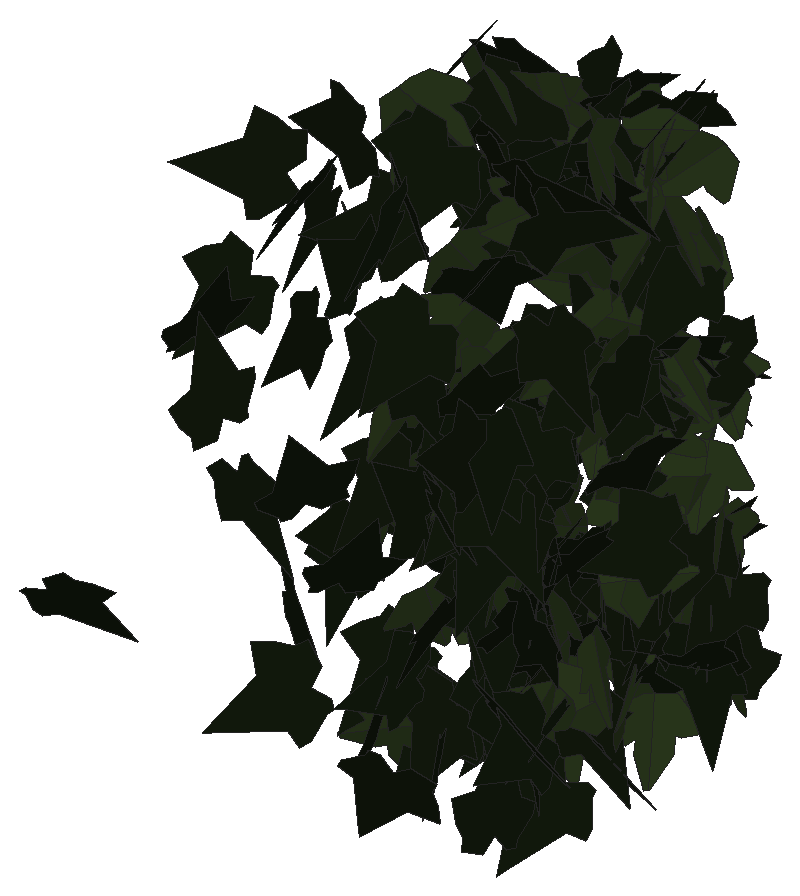
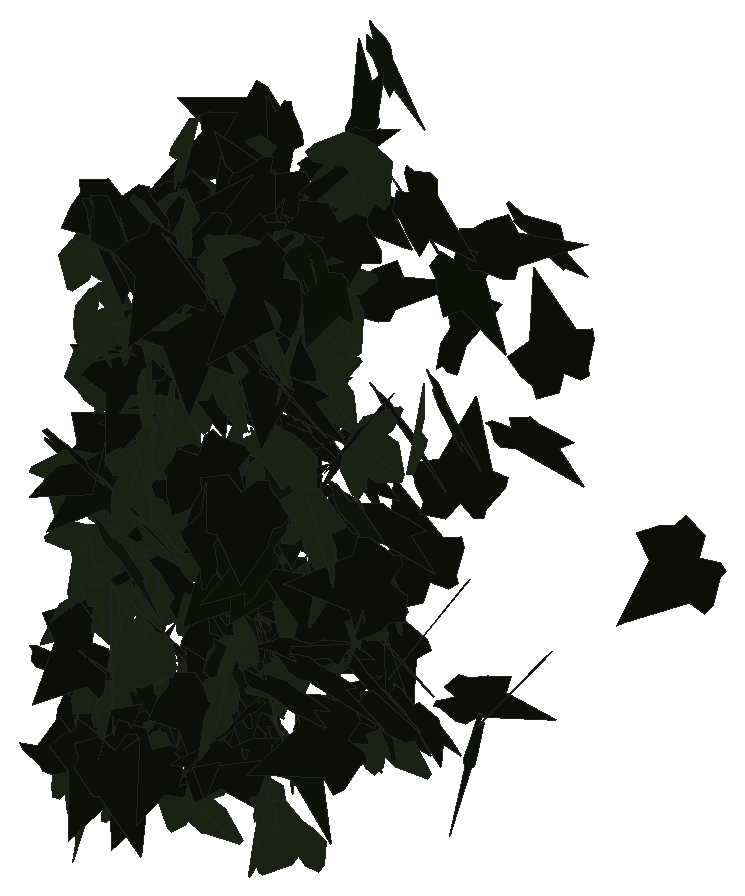
# SketchUp Ruby script. Lengths in inches.
U = 1.inch
M = Sketchup.active_model
def pt(a) = Geom::Point3d.new(a.map { |v| v * U })
def face(e, loops, mat)
  f = e.add_face(loops[0].map { |a| pt(a) })
  loops[1..].each { |l| e.add_face(l.map { |a| pt(a) }).erase! }
  f.material = f.back_material = mat if mat
  f
end
# faces: each face lists its corners as indices into pts; further lists are holes
def faces(e, pts, list, mat = nil) = list.each { |f| face(e, (f[0].is_a?(Array) ? f : [f]).map { |l| l.map { |i| pts[i] } }, mat) }
# xy, xz, yz: faces in a plane at the given z, y or x. An outline is a flat list of corners, or four numbers for a rectangle; further outlines are holes
def ring(l) = l.size == 4 ? [[l[0], l[1]], [l[2], l[1]], [l[2], l[3]], [l[0], l[3]]] : l.each_slice(2).to_a
def flat(e, list, mat, &to3) = list.each { |f| face(e, (f[0].is_a?(Array) ? f : [f]).map { |l| ring(l).map { |u, v| to3.(u, v) } }, mat) }
def xy(e, z, list, mat = nil) = flat(e, list, mat) { |x, y| [x, y, z] }
def xz(e, y, list, mat = nil) = flat(e, list, mat) { |x, z| [x, y, z] }
def yz(e, x, list, mat = nil) = flat(e, list, mat) { |y, z| [x, y, z] }
def lines(e, pts, list) = list.each { |a, b| e.add_line(pt(pts[a]), pt(pts[b])) }
# prism: a flat outline (further loops are holes) pulled along v
def prism(e, loops, v, mat = nil)
  f = face(e, loops, mat); d = Geom::Vector3d.new(v.map { |x| x * U })
  f.pushpull(f.normal.samedirection?(d) ? d.length : -d.length)
end
def box(e, o, s, mat = nil) = prism(e, [[o, [o[0] + s[0], o[1], o[2]], [o[0] + s[0], o[1] + s[1], o[2]], [o[0], o[1] + s[1], o[2]]]], [0, 0, s[2]], mat)
def at(x, y, z, deg = 0) = Geom::Transformation.translation(pt([x, y, z])) * Geom::Transformation.rotation(ORIGIN, Z_AXIS, deg.degrees)
def axes(o, x, y, z) = Geom::Transformation.new([*x, 0, *y, 0, *z, 0, *pt(o).to_a, 1])
def part(name) = M.definitions.add(name)
# library, detail: a bought-in or finely detailed component or shape, given as its bounding box
def library(name, o, s) = part(name).tap { |d| box(d.entities, o, s) }
def detail(e, o, s) = box(e.add_group.entities, o, s)
def put(e, d, t, mat = nil) = e.add_instance(d, t).tap { |i| i.material = mat if mat }
def group(e, t, mat = nil) = e.add_group.tap { |g| g.transformation = t; g.material = mat if mat }.entities
root = M.entities
M.materials.add("efeu1").color = [18, 25, 13]
M.materials.add("efeu2").color = [43, 57, 29]
c1 = part("ivyleaf_9")
p = [[1.54,2.16,1.25],[1.36,2.04,1.19],[-0.21,0.99,0.68],[-0.71,1.11,0.82],[-0.85,0.86,0.67],[-0.8,0.17,0.21],
  [-0.9,-0.01,0.1],[-0.67,-0.16,-0.02],[-0.08,-0.08,-0.05],[-0.03,-0.6,-0.4],[0.65,-0.88,-0.66],[0.83,-0.6,-0.49],
  [1.29,-0.42,-0.43],[1.8125,-0.07,-0.26],[1.21,0.44,0.15]]
faces(c1.entities,p,[[0,1,2,3,4,5,6,7,8,9,10,11,12,13,14]],"efeu1")
c2 = part("ivyleaf_10")
p = [[0,0.5,-0.03],[-0.0625,2.02,-0.43],[-0.19,2.01,-0.46],[-0.54,1.05,-0.29],[-0.52,0.625,-0.18],[-0.83,0.76,-0.28],
  [-1.16,0.64,-0.33],[-1.15,0.33,-0.24],[-0.77,-0.39,0.02],[-0.3,-0.51,0.16],[0.04,-0.48,0.23],[-0.02,2.01,-0.4375],
  [-0.06,2.01,-0.43],[0.04,-0.49,0.23],[0.67,-0.49,0.14],[1.38,0.36,-0.2],[1.375,0.51,-0.24],[0.81,0.65,-0.19],
  [0.62,0.59,-0.15],[0.6,1.09,-0.28],[0.5,1.23,-0.31]]
faces(c2.entities,p,[[0,1,2,3,4,5,6,7,8,9,10],[11,12,0,13,14,15,16,17,18,19,20]],"efeu2")
put(root,c1,axes([1.91,221.53,235.64],[0.22863,-0.36807,-0.09829],[-0.00412,0.10612,-0.43871],[0.41039,0.20612,0.05036]))
put(root,c1,axes([2.04,217.83,235.76],[0.42687,0.15912,0.09116],[0.08714,0.03428,-0.44312],[-0.17578,0.4034,0.0017]))
put(root,c1,axes([2.52,220.89,238.83],[-0.44623,-0.13584,0.00812],[-0.00782,-0.00297,-0.45233],[0.14674,-0.41324,0.00058]))
put(root,c1,axes([2.8,221.32,234.46],[0.2674,-0.1092,-0.35421],[-0.3342,0.14231,-0.28141],[0.1937,0.39629,0.00346]))
put(root,c1,axes([2.92,221.94,239.62],[-0.37271,0.12519,-0.2427],[0.23278,-0.08994,-0.38167],[-0.16618,-0.40677,0.0097]))
put(root,c1,axes([2.97,219.37,238.9],[0.24821,0.31767,0.19593],[-0.11941,-0.15254,0.40777],[0.38059,-0.25504,0.00015]))
put(root,c1,axes([3.48,220.34,240.84],[-0.23642,-0.04216,0.38848],[-0.38822,-0.10298,-0.23117],[0.11877,-0.42053,0.01766]))
put(root,c2,axes([3.16,222.16,238.78],[-0.2934,0.28026,0.19972],[0.14683,-0.13566,0.40592],[0.33626,0.30377,-0.00299]))
put(root,c1,axes([3.2,222.06,235.05],[-0.37672,-0.07268,-0.25952],[0.27137,0.01248,-0.36907],[0.07176,-0.4287,0.03325]))
put(root,c1,axes([3.34,222.51,237.02],[0.11116,0.25592,-0.34981],[0.04678,0.33797,0.28123],[0.45406,-0.09748,0.05666]))
put(root,c1,axes([3.74,220.55,240.65],[-0.23139,0.32472,-0.20241],[0.08986,-0.17778,-0.40373],[-0.39887,-0.22842,0.02647]))
put(root,c2,axes([3.6,222.6875,236.56],[-0.12476,0.29797,-0.30692],[0.07464,-0.2884,-0.33097],[-0.44674,-0.1314,0.03042]))
put(root,c1,axes([4.09,222.42,235.67],[-0.38619,0.23182,0.21706],[-0.18444,0.11449,-0.45042],[-0.25853,-0.42797,-0.00292]))
put(root,c1,axes([3.99,220.17,234.11],[-0.36444,-0.1518,0.23787],[-0.22521,-0.09397,-0.38482],[0.19282,-0.39667,0.00013]))
put(root,c1,axes([3.94,223.46,236.03],[-0.49598,-0.06285,-0.00765],[0.01361,-0.04677,-0.49762],[0.06184,-0.49382,0.0481]))
put(root,c1,axes([3.72,221.51,235.45],[0.19024,-0.34359,-0.20836],[0.09783,-0.17871,0.40156],[-0.41827,-0.19807,-0.00085]))
put(root,c1,axes([4.09,222.76,241.36],[0.04322,0.36416,0.24392],[-0.01197,0.23632,-0.37964],[-0.46765,0.02761,0.03226]))
put(root,c1,axes([4.35,220.7,241.51],[-0.11201,0.06327,-0.4344],[-0.43613,-0.14117,0.08204],[-0.13401,0.40656,0.09609]))
put(root,c2,axes([4.21,223,237.99],[-0.44215,0.05122,0.22777],[-0.23326,-0.07694,-0.43551],[-0.00956,-0.49138,0.09194]))
put(root,c1,axes([3.7,222.91,234.78],[0.4087,0.06535,0.21249],[0.21981,0.02155,-0.3992],[-0.07321,0.42952,-0.0123]))
put(root,c2,axes([4.15,223.84,234.18],[0.0767,-0.37169,-0.32552],[0.00816,0.33032,-0.37526],[0.49402,0.05225,0.05673]))
put(root,c2,axes([4.13,222.73,236.99],[-0.1661,0.42601,-0.2023],[-0.0532,-0.23004,-0.44074],[-0.4686,-0.12489,0.12174]))
put(root,c2,axes([3.875,223.66,233.75],[0.38828,0.08163,0.30426],[0.28914,0.09934,-0.39563],[-0.12505,0.48318,0.02994]))
put(root,c1,axes([3.79,222.85,236.47],[0.32966,0.15313,-0.28023],[0.25976,0.12146,0.35516],[0.21109,-0.38862,0.00059]))
put(root,c1,axes([4.18,219.93,236.82],[0.28208,0.17465,0.31287],[-0.26574,-0.17317,0.32672],[0.26557,-0.35879,-0.00539]))
put(root,c1,axes([4.35,223.59,235.6875],[-0.46956,-0.13976,-0.09989],[0.11476,-0.03884,-0.4851],[0.12784,-0.4785,0.06855]))
put(root,c1,axes([4.08,223.11,236.13],[-0.19881,-0.41807,-0.18891],[0.22689,0.08934,-0.43651],[0.39874,-0.25929,0.15419]))
put(root,c2,axes([4.25,221.4,236.43],[0.40162,-0.29312,0.05273],[0.04132,-0.03283,-0.49721],[0.29494,0.40374,-0.00215]))
put(root,c1,axes([4.47,221.03,238.55],[-0.46847,0.10262,-0.14145],[0.14112,-0.01654,-0.47939],[-0.10307,-0.48908,-0.01347]))
put(root,c1,axes([4.625,221.57,237.26],[-0.23945,0.33896,0.16501],[-0.10902,0.12342,-0.42091],[-0.38922,-0.2431,0.01638]))
put(root,c2,axes([4.63,223.45,240.74],[0.17537,-0.15369,-0.4423],[-0.33914,0.28395,-0.23314],[0.32284,0.38177,-0.00465]))
put(root,c1,axes([4.29,219.94,239.28],[0.00885,-0.14754,-0.4255],[0.29714,-0.31517,0.12393],[-0.36379,-0.26101,0.09087]))
put(root,c2,axes([4.44,222.98,240.4],[-0.23147,0.3678,0.0931],[-0.04652,0.07851,-0.44271],[-0.40616,-0.2186,-0.00235]))
put(root,c1,axes([4.58,221.36,234.32],[-0.4209,-0.19256,0.01681],[-0.01592,-0.00666,-0.45209],[0.20808,-0.39,-0.00058]))
put(root,c1,axes([4.71,221.2,240.11],[-0.24158,-0.08892,0.37683],[-0.34095,-0.18003,-0.24863],[0.21473,-0.38589,0.02916]))
put(root,c2,axes([4.87,220.82,233.63],[-0.18329,-0.03834,0.41464],[-0.41276,-0.11405,-0.1806],[0.12942,-0.41803,0.01124]))
put(root,c2,axes([4.73,222.09,240.66],[-0.30498,-0.30563,0.25215],[-0.17014,-0.18634,-0.43166],[0.35782,-0.3491,0.00966]))
put(root,c2,axes([4.68,222.72,241.46],[-0.45211,0.17823,0.11761],[-0.13564,-0.02701,-0.48049],[-0.16493,-0.46637,0.07277]))
put(root,c1,axes([4.72,221.13,236.91],[-0.44715,-0.13343,-0.002],[0.00182,0.00104,-0.4524],[0.14411,-0.41403,-0.00049]))
put(root,c1,axes([4.38,223.36,241.43],[0.49307,0.08084,-0.01864],[-0.01555,-0.02027,-0.49935],[-0.08149,0.49301,-0.01747]))
put(root,c1,axes([4.86,217.5,239.3],[-0.44645,0.07294,-0.11869],[-0.12498,0.00024,0.4361],[0.07601,0.42884,0.01994]))
put(root,c1,axes([4.47,220.24,235.71],[0.33519,0.27585,0.13483],[-0.10596,-0.08477,0.43184],[0.31166,-0.3255,0.0018]))
put(root,c1,axes([4.88,222.96,239.58],[-0.47782,-0.14516,0.02476],[-0.02349,-0.00787,-0.49939],[0.14537,-0.4784,0.00071]))
put(root,c2,axes([4.71,221.27,237.97],[-0.04403,-0.33624,0.36743],[0.0614,-0.36971,-0.33097],[0.49426,0.01598,0.07385]))
put(root,c1,axes([4.74,221.73,241.37],[0.29999,0.28944,-0.17494],[-0.1364,-0.11182,-0.417],[-0.33483,0.30487,0.01313]))
put(root,c1,axes([5.03,223.16,240.08],[-0.45458,0.19879,0.06197],[-0.05888,0.02002,-0.49612],[-0.19973,-0.45835,0.00521]))
put(root,c2,axes([4.81,222.58,236.24],[0.00958,-0.13557,0.42977],[-0.00025,-0.41333,-0.14101],[0.4697,0.00254,-0.00884]))
put(root,c1,axes([4.69,220.49,233.45],[0.0285,0.30612,0.32024],[-0.06786,-0.30256,0.31841],[0.464,-0.06305,0.0269]))
put(root,c1,axes([4.54,223.35,237.43],[0.41422,-0.2796,-0.01559],[0.0049,0.03508,-0.49874],[0.27999,0.41303,0.03181]))
put(root,c1,axes([4.88,222.89,240.1],[0.22329,0.36146,-0.13082],[-0.0561,-0.11514,-0.43291],[-0.40952,0.21286,-0.01202]))
put(root,c1,axes([4.68,221.28,238.26],[0.25092,-0.38907,-0.18885],[-0.08712,0.16839,-0.46266],[0.42361,0.26509,0.01672]))
put(root,c2,axes([4.93,223.63,235.875],[-0.28292,0.30763,0.16758],[-0.10194,0.13117,-0.42002],[-0.36094,-0.27818,-0.01273]))
put(root,c2,axes([5.05,223.58,235.17],[-0.00151,0.18181,0.41099],[-0.18354,0.36355,-0.17458],[-0.43246,-0.15492,0.07266]))
put(root,c1,axes([5.24,222.14,237.59],[-0.20989,0.36517,0.13994],[-0.09032,0.1077,-0.4296],[-0.41049,-0.21041,0.02297]))
put(root,c1,axes([5.18,223.64,234.54],[-0.12312,0.28985,-0.31582],[-0.03229,-0.31948,-0.30546],[-0.45223,-0.0561,0.10779]))
put(root,c1,axes([5.22,221.98,233.77],[-0.21082,0.3885,-0.01428],[0.00384,-0.01358,-0.45216],[-0.41982,-0.19522,0.00303]))
put(root,c1,axes([5.32,219.46,240.38],[-0.15963,0.24995,0.33685],[-0.1875,0.27352,-0.30191],[-0.40009,-0.2279,0.00709]))
put(root,c1,axes([5.14,223.17,237.93],[0.24959,0.27867,-0.25082],[-0.19043,-0.16636,-0.37564],[-0.34951,0.28964,0.02556]))
put(root,c2,axes([5.03,220.85,241.36],[-0.04364,0.36744,0.33628],[-0.02524,0.3355,-0.36987],[-0.49745,-0.04926,-0.01074]))
put(root,c2,axes([5.25,221.63,238.98],[-0.23345,-0.26805,0.27643],[-0.16532,-0.21774,-0.35783],[0.37267,-0.2645,0.01443]))
put(root,c1,axes([5.32,221.51,236.8125],[-0.18239,0.08143,-0.40822],[-0.37409,0.18478,0.19485],[0.21795,0.38529,-0.00717]))
put(root,c2,axes([5.08,221.1,235.35],[-0.19617,-0.36509,-0.15754],[0.07411,0.13505,-0.42408],[0.4204,-0.19416,0.00125]))
put(root,c1,axes([4.84,223.78,234.625],[0.05969,-0.39616,-0.29916],[0.10371,0.30462,-0.38269],[0.48547,-0.01637,0.11853]))
put(root,c2,axes([4.92,221.07,242.01],[-0.32586,-0.19515,-0.32516],[0.31837,0.09216,-0.37437],[0.20605,-0.45103,0.06419]))
put(root,c2,axes([5.1,221.63,239.79],[-0.15753,-0.31569,-0.27178],[0.13259,0.23098,-0.36147],[0.42227,-0.1903,0.01211]))
put(root,c1,axes([5.07,222.93,241.33],[-0.15838,-0.47345,0.02749],[0.00782,-0.03158,-0.49894],[0.47419,-0.15762,0.0174]))
put(root,c2,axes([5.12,222.11,234.875],[0.01544,-0.03948,0.45029],[-0.0226,0.43264,0.04175],[-0.469,-0.02215,0.01281]))
put(root,c2,axes([5.2,223.08,241.39],[-0.43157,-0.16053,-0.06391],[0.06028,0.0259,-0.44785],[0.17558,-0.40347,-0.00332]))
put(root,c1,axes([5.28,222.17,237.3],[-0.29199,0.16134,-0.31217],[0.19879,-0.25332,-0.31403],[-0.30973,-0.31468,0.09274]))
put(root,c1,axes([5,223.68,234.77],[0.11581,-0.48628,-0.01094],[-0.00117,0.01096,-0.49988],[0.4864,0.1158,0.0014]))
put(root,c1,axes([5.52,220.26,234.75],[-0.39538,0.21231,0.10463],[-0.10056,0.0399,-0.43996],[-0.23296,-0.37757,0.01234]))
put(root,c1,axes([5.43,222.83,235.12],[-0.0572,0.39888,0.17188],[-0.04856,0.1605,-0.41787],[-0.46377,-0.066,0.02256]))
put(root,c2,axes([5.5,223.28,239.78],[-0.36754,0.04791,0.27734],[-0.29262,-0.05965,-0.34845],[-0.00036,-0.42822,0.07956]))
put(root,c1,axes([5.375,221.24,233.83],[-0.42914,-0.17571,-0.02237],[0.01695,0.01767,-0.45173],[0.19043,-0.39754,-0.01019]))
put(root,c1,axes([5.08,221.12,241.73],[0.10355,-0.30357,-0.3083],[-0.01198,0.30202,-0.32538],[0.45809,0.07652,0.06118]))
put(root,c2,axes([5.54,223.85,233.78],[0.27974,0.06517,-0.35708],[-0.37518,0.00135,-0.27228],[-0.04121,0.43009,0.05496]))
put(root,c2,axes([5.15,222.24,238.15],[-0.3425,-0.12224,-0.28236],[0.28072,0.07982,-0.35313],[0.15685,-0.40977,0.01545]))
put(root,c1,axes([5.41,223.55,235.11],[0.14136,0.40087,-0.11102],[-0.03896,-0.10051,-0.43856],[-0.44633,0.13574,0.00312]))
put(root,c1,axes([5.71,220.22,237.03],[-0.26667,0.04086,-0.37002],[-0.38652,-0.01243,0.25683],[0.01408,0.4329,0.0423]))
put(root,c1,axes([5.73,222.35,240.36],[-0.34248,0.01657,-0.3092],[-0.32056,-0.05237,0.32621],[-0.02575,0.43152,0.05146]))
put(root,c1,axes([5.46,222.36,236.5625],[0.0923,0.33542,0.27401],[0.00335,0.26821,-0.35616],[-0.46063,0.06916,0.05231]))
put(root,c2,axes([5.11,223.04,241.14],[0.25833,0.09763,0.41681],[0.2611,0.34987,-0.24377],[-0.33925,0.3436,0.12978]))
put(root,c2,axes([5.22,222.18,233.77],[-0.13995,0.00138,-0.43186],[0.21283,-0.38269,-0.06527],[-0.39475,-0.20681,0.11791]))
put(root,c1,axes([5.47,223.36,237.21],[0.02405,-0.00157,0.4518],[0.10914,0.42308,-0.0038],[-0.45631,0.10111,0.0229]))
put(root,c1,axes([5.43,221.14,233.92],[-0.17635,-0.37956,0.14144],[-0.03736,-0.13299,-0.42923],[0.43384,-0.16574,0.02052]))
put(root,c1,axes([5.64,221.91,234.5],[0.04317,0.02492,0.44974],[-0.03082,0.43349,-0.02323],[-0.4668,-0.02631,0.04313]))
put(root,c1,axes([5.67,223.55,240.6],[0.29569,0.24859,-0.23823],[-0.19094,-0.14594,-0.38448],[-0.31117,0.32577,0.00955]))
put(root,c1,axes([5.75,220.3125,233.3],[0.00224,0.08388,0.4439],[-0.0298,0.426,-0.08693],[-0.46885,-0.02668,0.00764]))
put(root,c1,axes([5.88,222.49,236.2],[-0.1521,0.31082,0.28057],[-0.15134,0.23189,-0.35393],[-0.41794,-0.19709,0.02605]))
put(root,c1,axes([5.64,220.73,241.7],[-0.25264,-0.41632,0.11335],[-0.05836,-0.09718,-0.48698],[0.42751,-0.25929,0.00051]))
put(root,c1,axes([5.62,222.68,236.53],[0.18904,0.3088,0.26151],[0.05885,0.25351,-0.36324],[-0.42604,0.17204,0.06586]))
put(root,c1,axes([5.82,221.97,233.93],[-0.45898,0.00515,-0.09638],[0.09986,-0.01399,-0.44182],[-0.00865,-0.43474,0.01307]))
put(root,c1,axes([5.83,223.15,238.23],[-0.03944,0.27405,-0.34927],[0.01398,-0.33619,-0.28678],[-0.46793,-0.03314,0.02088]))
put(root,c1,axes([5.85,223.63,241.46],[-0.44152,0.10751,-0.10676],[0.11059,-0.01407,-0.43944],[-0.11637,-0.42127,-0.01256]))
put(root,c1,axes([5.62,222.42,237.76],[-0.06557,0.07534,-0.44107],[0.32515,-0.29889,-0.10004],[-0.33271,-0.30694,-0.01084]))
put(root,c1,axes([5.94,219.35,233.99],[0.21202,0.19552,-0.34876],[-0.26726,-0.2265,-0.288],[-0.323,0.31575,0.00937]))
put(root,c2,axes([5.84,222.24,234.9],[0.11751,-0.21115,0.379],[-0.10715,0.35294,0.24349],[-0.44207,-0.14168,0.04172]))
put(root,c1,axes([5.75,221.5,235.64],[-0.09905,-0.42373,0.03702],[0.01487,-0.03935,-0.45032],[0.459,-0.09016,0.02258]))
put(root,c1,axes([5.9375,221.5,236.93],[-0.23178,-0.30534,0.2324],[-0.11068,-0.2004,-0.38713],[0.39337,-0.23629,0.02801]))
put(root,c2,axes([5.83,223.47,234.96],[-0.20402,0.31232,-0.24609],[0.04111,-0.24682,-0.37041],[-0.42119,-0.17538,0.08305]))
put(root,c1,axes([5.87,223.59,241.29],[0.24421,0.36146,0.08973],[0.05361,0.07071,-0.44339],[-0.39774,0.23146,-0.00467]))
put(root,c2,axes([5.92,223.68,239.13],[-0.07899,0.33866,-0.27355],[-0.05702,-0.27191,-0.34883],[-0.45959,-0.02447,0.0903]))
put(root,c1,axes([5.57,221.46,236.79],[0.32295,-0.21634,0.23944],[0.20522,-0.1301,-0.3838],[0.27259,0.35425,0.00527]))
put(root,c1,axes([6.07,222.95,239.83],[0.0448,0.37122,-0.23185],[-0.04951,-0.21893,-0.38801],[-0.46503,0.05907,0.01897]))
put(root,c2,axes([5.93,223.7,240.36],[0.3925,0.23466,-0.04749],[-0.0377,-0.03011,-0.44985],[-0.25542,0.36504,-0.00658]))
put(root,c2,axes([6.06,223.76,239.08],[-0.45798,-0.09439,0.02312],[-0.02183,-0.01147,-0.45175],[0.10243,-0.42448,0.00706]))
put(root,c1,axes([5.98,224,234.26],[0.35182,0.27689,-0.08347],[-0.07877,-0.03801,-0.44424],[-0.30122,0.33334,0.01868]))
put(root,c2,axes([6.15,221.6,235.62],[0.1263,-0.0899,0.4256],[-0.26186,0.33198,0.14791],[-0.36904,-0.26634,0.0407]))
put(root,c1,axes([5.92,221.53,234.25],[-0.06738,-0.43043,0.00826],[-0.01371,-0.00618,-0.45216],[0.46474,-0.06259,-0.01214]))
put(root,c1,axes([6.3,221.89,234.61],[-0.36729,0.26784,0.04448],[-0.03577,0.02708,-0.45021],[-0.29074,-0.34169,-0.00081]))
put(root,c1,axes([6.17,220.1,236.01],[-0.20603,0.31121,-0.24606],[0.12032,-0.20907,-0.37943],[-0.40471,-0.22059,0.01247]))
put(root,c1,axes([6.375,221.54,238.93],[-0.37103,0.25783,0.0715],[-0.07274,0.02467,-0.44621],[-0.27885,-0.34949,0.02125]))
put(root,c1,axes([6.25,222.96,240],[-0.17382,0.3651,-0.18019],[0.06697,-0.16198,-0.41489],[-0.43129,-0.1723,0.0082]))
put(root,c2,axes([6.16,221.07,236.15],[0.21435,-0.36944,-0.25993],[-0.05958,0.26208,-0.42162],[0.44778,0.21173,0.06834]))
put(root,c1,axes([6.26,224.34,234.29],[0.01182,0.39579,-0.18737],[-0.02216,-0.17955,-0.41151],[-0.46913,0.01845,0.01472]))
put(root,c2,axes([6.18,223.77,239.4],[0.12172,-0.41864,-0.03702],[-0.01509,0.0331,-0.45085],[0.45351,0.11346,-0.00507]))
put(root,c1,axes([6.51,221.47,235.34],[-0.08811,0.14345,0.41858],[-0.39356,0.19059,-0.14747],[-0.24096,-0.36376,0.0878]))
put(root,c2,axes([6.18,221.41,237.46],[0.39399,-0.23174,-0.05139],[-0.04663,0.02419,-0.44946],[0.25162,0.36734,-0.00282]))
put(root,c1,axes([6.08,221.15,235.6875],[-0.28024,-0.2547,-0.24834],[0.18485,0.1665,-0.37814],[0.32864,-0.31085,0.00093]))
put(root,c2,axes([6.28,223.93,238.26],[0.03347,0.24344,0.37353],[-0.20083,0.33279,-0.2179],[-0.42339,-0.13861,0.13289]))
put(root,c1,axes([5.99,219.63,241.47],[-0.04265,-0.07224,0.44422],[0.13032,-0.41377,-0.06118],[0.44934,0.11314,0.05991]))
put(root,c1,axes([6.23,220.57,240.34],[0.25368,0.35829,-0.07838],[-0.04784,-0.06107,-0.44554],[-0.39252,0.23901,0.00365]))
put(root,c1,axes([6.49,221.55,236.6],[0.04493,0.03808,-0.44858],[-0.46759,-0.00278,-0.04369],[-0.00695,0.43332,0.03914]))
put(root,c2,axes([6.21,222.875,239.9375],[0.43386,0.15162,-0.07249],[-0.06944,-0.02703,-0.44655],[-0.16631,0.40682,-0.00266]))
put(root,c2,axes([6.07,224.02,235.88],[0.40696,0.13573,0.17653],[0.13001,0.15252,-0.40476],[-0.19543,0.38411,0.09834]))
put(root,c2,axes([6.28,222.04,237.1],[-0.46019,0.08632,0.01515],[0.01369,-0.01075,0.45207],[0.09355,0.42621,0.00834]))
put(root,c1,axes([6.44,220.74,240.49],[-0.14857,0.41252,0.01153],[-0.00475,0.01022,-0.45225],[-0.44566,-0.13764,0.00098]))
put(root,c1,axes([6.36,219.45,240.125],[-0.37965,-0.25422,0.03324],[-0.0309,-0.01497,-0.45115],[0.27499,-0.35266,-0.00481]))
put(root,c1,axes([6.46,220.5,237.43],[-0.46569,-0.05654,0.0102],[-0.01023,-0.00319,-0.45228],[0.06112,-0.4313,0.00201]))
put(root,c1,axes([6.17,219.9,237.54],[0.38728,-0.15387,-0.19994],[-0.17834,0.10167,-0.40496],[0.19728,0.39397,0.02641]))
put(root,c1,axes([6.38,221.74,241.25],[-0.01648,-0.10639,-0.43837],[0.11336,-0.4102,0.10372],[-0.45562,-0.09821,0.04166]))
put(root,c1,axes([6.19,223.73,234.41],[-0.07825,-0.45622,0.18906],[0.04707,-0.19744,-0.45695],[0.49159,-0.05371,0.07385]))
put(root,c1,axes([6.63,221.4,237.1],[-0.06836,0.27861,0.34114],[-0.23621,0.26472,-0.27773],[-0.4003,-0.20378,0.10563]))
put(root,c2,axes([6.4,221.16,236.24],[-0.05191,-0.43137,0.03008],[-0.00183,-0.02892,-0.4514],[0.46692,-0.04807,0.00157]))
put(root,c1,axes([6.64,223.85,237.02],[-0.239,0.31731,0.20687],[-0.13729,0.15368,-0.40205],[-0.38045,-0.25479,0.01513]))
put(root,c2,axes([6.54,221.72,233.75],[0.35586,-0.00558,-0.2953],[-0.30509,0.03835,-0.3417],[0.03159,0.43327,0.02644]))
put(root,c1,axes([6.4375,224.42,234.22],[0.10026,0.38725,0.18207],[0.03176,0.17291,-0.414],[-0.45788,0.09679,0.01115]))
put(root,c1,axes([6.5,221.77,234.89],[0.05489,0.41678,-0.11828],[-0.01427,-0.11296,-0.43666],[-0.46636,0.05251,-0.00056]))
put(root,c1,axes([6.58,223.67,238.74],[-0.41313,-0.16673,0.12781],[-0.10925,-0.07484,-0.43306],[0.1952,-0.39475,0.02812]))
put(root,c1,axes([6.53,218.6875,242.04],[-0.35881,0.21462,-0.1883],[0.16725,-0.09393,-0.41132],[-0.25297,-0.36652,-0.00485]))
put(root,c1,axes([6.2,221.125,240.85],[-0.2099,0.04791,0.40166],[0.40565,-0.08989,0.20817],[0.11,0.42291,-0.00125]))
put(root,c1,axes([6.24,221.38,234.04],[0.03283,-0.4919,0.08338],[0.00678,-0.08311,-0.493],[0.49888,0.0335,0.00122]))
put(root,c2,axes([6.43,224.15,236.34],[0.26392,-0.32652,-0.15736],[0.00257,0.18436,-0.40975],[0.38866,0.2205,0.10957]))
put(root,c1,axes([6.5625,220.71,241.87],[0.27757,0.04336,-0.3622],[-0.37277,-0.0469,-0.27098],[-0.06861,0.43028,0.00697]))
put(root,c1,axes([6.28,221.6875,240.34],[0.40114,0.19025,0.12767],[-0.12752,-0.03849,0.43357],[0.20865,-0.38929,0.01953]))
put(root,c1,axes([6.43,223.53,239.47],[0.36791,0.2556,-0.09215],[-0.10966,-0.01126,-0.43975],[-0.2708,0.35181,0.05288]))
put(root,c2,axes([6.67,222.59,241.31],[-0.35742,0.10941,0.27066],[-0.26655,0.08257,-0.36251],[-0.14803,-0.41284,-0.00077]))
put(root,c1,axes([6.28,220.24,238.62],[0.13831,0.03219,0.43105],[0.33454,0.28185,-0.1223],[-0.29944,0.32977,0.06246]))
put(root,c2,axes([6.3125,222.65,238.93],[-0.1568,-0.14995,-0.39692],[0.28648,0.27441,-0.21707],[0.33772,-0.30239,-0.00015]))
put(root,c2,axes([6.31,222.93,240.57],[0.41784,0.13558,0.15129],[0.14857,0.04733,-0.42635],[-0.15509,0.41061,-0.00081]))
put(root,c2,axes([6.5,224.26,234.74],[-0.29637,0.33735,0.01131],[-0.02671,-0.00612,-0.45162],[-0.36355,-0.27456,0.02397]))
put(root,c1,axes([6.39,222.54,240.44],[0.2346,-0.233,-0.30808],[-0.17736,0.24923,-0.32911],[0.36636,0.26986,0.03795]))
put(root,c1,axes([6.41,220.85,235.5],[0.20013,0.28112,0.28644],[0.17242,0.22456,-0.35008],[-0.3885,0.24448,-0.00781]))
put(root,c2,axes([6.44,222.64,237.74],[0.379,0.25615,-0.02234],[-0.01687,-0.01504,-0.45184],[-0.2771,0.35126,-0.00305]))
put(root,c2,axes([6.47,221.61,235.87],[-0.11554,0.25902,-0.34601],[0.02873,-0.33841,-0.2829],[-0.45446,-0.08725,0.07009]))
put(root,c1,axes([6.64,220.36,237.76],[-0.33889,-0.28755,0.09344],[-0.0719,-0.06034,-0.44264],[0.31732,-0.32078,-0.0005]))
put(root,c2,axes([6.62,224.38,233.66],[-0.21733,0.30108,0.25065],[-0.14057,0.20287,-0.3766],[-0.39207,-0.23962,-0.00391]))
put(root,c1,axes([6.75,221.3,234.98],[-0.17997,0.40151,-0.01637],[-0.00003,-0.01705,-0.45205],[-0.43396,-0.16651,0.00682]))
put(root,c1,axes([6.51,222,233.8],[-0.07543,-0.22243,0.38194],[0.27782,0.27623,0.22487],[-0.37127,0.25189,0.09067]))
put(root,c1,axes([6.72,222.57,240.85],[-0.08208,0.03174,0.44422],[-0.34851,-0.28949,-0.03734],[0.30416,-0.32313,0.07709]))
put(root,c2,axes([6.79,220.82,241.24],[0.29377,-0.07894,-0.34337],[-0.33195,0.12234,-0.29377],[0.15564,0.40991,0.02155]))
put(root,c1,axes([6.39,220.65,238.37],[0.04004,-0.49033,0.08927],[0.02124,-0.0878,-0.49177],[0.49794,0.04318,0.0138]))
put(root,c1,axes([6.59,220.07,238.12],[-0.05697,-0.05389,0.44555],[-0.18794,-0.39234,-0.07361],[0.42678,-0.17997,0.02706]))
put(root,c2,axes([6.4375,221.91,234.4],[0.44747,-0.04058,0.13118],[0.13745,0.00665,-0.43255],[0.03982,0.43305,0.01893]))
put(root,c2,axes([6.93,221.84,239.83],[0.09136,0.01866,-0.44334],[-0.45667,0.06192,-0.08445],[0.06177,0.43017,0.03138]))
put(root,c1,axes([6.6,223.16,236.47],[-0.37693,-0.14901,-0.22114],[0.22774,0.0452,-0.39289],[0.16362,-0.40617,0.03741]))
put(root,c1,axes([6.56,223.22,240.17],[-0.16089,-0.40073,-0.0835],[0.02756,0.07616,-0.44462],[0.44053,-0.15112,-0.00267]))
put(root,c2,axes([6.78,223.74,234.29],[0.1121,-0.25311,-0.35174],[-0.14309,0.31119,-0.2845],[0.43321,0.16829,-0.00295]))
put(root,c2,axes([6.71,221.4,235.73],[-0.42118,0.18762,0.04583],[-0.04275,0.01937,-0.45007],[-0.2037,-0.39198,-0.00031]))
put(root,c1,axes([6.51,222.37,240.0625],[-0.03337,-0.34655,0.27154],[0.04707,-0.26292,-0.35756],[0.46624,0.00174,0.05553]))
put(root,c2,axes([6.69,222.35,238.4],[0.22791,-0.38027,-0.00967],[-0.00317,0.009,-0.45229],[0.4108,0.21104,0.00187]))
put(root,c2,axes([6.61,222.82,236.61],[-0.02481,-0.38675,0.2057],[0.01171,0.19749,0.40293],[-0.469,0.02539,-0.00082]))
put(root,c1,axes([6.92,223.6875,237.68],[-0.45222,0.11766,-0.00746],[0.00009,-0.0262,-0.45158],[-0.12731,-0.41797,0.02621]))
put(root,c1,axes([6.71,223.47,238],[-0.27456,-0.32604,0.14066],[-0.03696,-0.14313,-0.42572],[0.37942,-0.24988,0.06032]))
put(root,c2,axes([6.59,223.03,236.39],[0.35777,0.28106,0.02295],[0.01799,0.01447,-0.45182],[-0.30395,0.33169,0.00027]))
put(root,c1,axes([6.71,220.33,237.09],[-0.40119,-0.15525,-0.17129],[0.1825,0.02036,-0.41633],[0.16263,-0.40584,0.04464]))
put(root,c1,axes([6.82,221.6,236.26],[-0.0207,0.41488,-0.13453],[0.01978,-0.1286,-0.43176],[-0.46893,-0.02374,-0.01227]))
put(root,c2,axes([6.71,221.625,239],[0.04132,0.15111,-0.42236],[-0.08731,-0.39804,-0.16196],[-0.45976,0.08917,-0.00721]))
put(root,c2,axes([6.71,223.48,237.68],[-0.44073,0.14833,-0.02733],[0.03048,0.00074,-0.45145],[-0.15981,-0.40893,-0.01073]))
put(root,c2,axes([6.8,221.29,234.34],[-0.10801,-0.25072,0.35476],[-0.03069,-0.34574,-0.27295],[0.45618,-0.08263,0.06563]))
put(root,c1,axes([6.72,221.15,238.05],[-0.26326,-0.36026,-0.00452],[0.00321,0.00324,-0.45238],[0.3891,-0.24378,0.00067]))
put(root,c2,axes([6.88,220.81,236.55],[-0.25455,0.2488,0.27861],[-0.20672,0.1876,-0.35633],[-0.33643,-0.30353,0.00814]))
put(root,c1,axes([6.85,222.15,238.45],[-0.35172,-0.2757,0.08798],[-0.05566,-0.06991,-0.44329],[0.30644,-0.32913,0.02047]))
put(root,c1,axes([6.95,223.39,241.46],[-0.15315,0.41105,0.01289],[-0.00346,0.012,-0.45222],[-0.44412,-0.14184,-0.00092]))
put(root,c2,axes([6.75,223.375,233.7],[-0.23749,-0.31962,-0.20463],[0.11745,0.164,-0.40346],[0.38796,-0.2453,-0.00311]))
put(root,c1,axes([6.86,220.96,233.91],[0.17078,-0.10225,-0.40782],[-0.36723,0.19551,-0.19562],[0.23809,0.3749,-0.00921]))
put(root,c2,axes([6.92,220.96,234.15],[-0.05419,0.08448,0.44071],[-0.21175,0.37571,-0.10205],[-0.41586,-0.20231,-0.00547]))
put(root,c1,axes([6.61,222.12,241.09],[0.4569,0.10008,0.01577],[0.01661,0.00085,-0.45212],[-0.10805,0.42333,-0.00282]))
put(root,c2,axes([6.95,221.83,234.23],[-0.10699,-0.06365,0.43551],[-0.10267,-0.41575,-0.08911],[0.44578,-0.11103,0.084]))
put(root,c1,axes([6.51,222.0625,233.62],[0.43042,-0.1523,0.08822],[0.08826,-0.02377,-0.44366],[0.16632,0.40677,0.00711]))
put(root,c1,axes([7.06,224.03,233.875],[0.14159,-0.11059,0.41575],[-0.35287,0.23073,0.17782],[-0.27595,-0.35179,-0.01407]))
put(root,c2,axes([6.71,223.37,233.92],[0.35944,0.27272,0.06646],[0.0577,0.03561,-0.44744],[-0.29696,0.33701,-0.0065]))
put(root,c1,axes([7,223.05,234.74],[-0.32988,0.2768,-0.14452],[0.11883,-0.08547,-0.42857],[-0.31268,-0.32451,-0.0104]))
put(root,c2,axes([6.78,222.9,239.78],[0.02492,-0.19768,0.40228],[0.13412,-0.36818,-0.20339],[0.44956,0.1208,0.03838]))
put(root,c2,axes([6.88,223.72,236.28],[-0.00665,0.19158,-0.40611],[0.00841,0.39052,0.19913],[0.46968,-0.00428,-0.00931]))
put(root,c1,axes([7.03,220.67,235.86],[0.19968,0.02658,-0.40857],[-0.42007,-0.0552,-0.19426],[-0.06617,0.43066,0.00031]))
put(root,c2,axes([6.9,223.32,241.25],[0.22903,-0.37195,-0.07995],[-0.04755,0.06337,-0.44522],[0.40743,0.21648,-0.00702]))
put(root,c2,axes([6.92,223.66,234.96],[-0.23205,-0.43835,0.06327],[0.0047,-0.07386,-0.49449],[0.44287,-0.2289,0.0384]))
put(root,c1,axes([6.97,223.34,241.67],[0.23255,0.32355,-0.20321],[-0.12463,-0.15786,-0.40411],[-0.38872,0.24418,0.008]))
put(root,c1,axes([7.19,222.43,234.97],[-0.01717,0.23413,0.38092],[-0.28743,0.28456,-0.20119],[-0.37122,-0.23116,0.13816]))
put(root,c2,axes([6.85,223.23,240.91],[-0.06707,0.37685,-0.21654],[-0.00247,-0.21065,-0.39581],[-0.46498,-0.05324,0.03334]))
put(root,c2,axes([7.12,223.7,239.1],[0.20081,0.19161,0.35716],[-0.25664,-0.24793,0.27767],[0.33841,-0.30173,-0.00136]))
put(root,c1,axes([6.79,223.14,234.76],[-0.08405,-0.20642,0.38991],[0.03278,-0.38276,-0.21262],[0.46106,-0.01042,0.08619]))
put(root,c1,axes([6.69,223.79,238.09],[0.46448,-0.06245,-0.01967],[-0.01986,0.00502,-0.45197],[0.06762,0.43046,0.00241]))
put(root,c2,axes([7.12,224.17,233.73],[-0.34909,0.17504,0.24191],[-0.24112,0.07399,-0.38057],[-0.20176,-0.39129,0.03625]))
put(root,c1,axes([7.17,220.61,234.33],[-0.19265,0.38984,0.07661],[-0.04804,0.0606,-0.44559],[-0.42578,-0.18323,0.01561]))
put(root,c1,axes([6.99,219.98,233.33],[-0.17353,-0.24497,0.33442],[0.22429,0.24685,0.30349],[-0.37456,0.26131,0.0268]))
put(root,c1,axes([7.17,220.52,237.34],[-0.46411,0.06544,-0.01727],[0.01774,-0.00243,-0.45207],[-0.07072,-0.43004,-0.00007]))
put(root,c1,axes([7.19,223.35,241.36],[-0.25936,0.36259,0.0092],[-0.00456,0.00782,-0.45231],[-0.39169,-0.24019,-0.00083]))
put(root,c2,axes([7.26,221.39,240.66],[-0.29896,-0.00869,0.34886],[-0.36238,0.00252,-0.2879],[0.00388,-0.43491,-0.00864]))
put(root,c2,axes([6.61,223.2,241.27],[0.141,-0.08071,-0.4233],[0.42156,-0.12088,0.15514],[-0.15204,-0.41,0.03759]))
put(root,c1,axes([6.82,221.92,234.11],[0.11822,-0.36571,-0.21691],[-0.05656,0.202,-0.39694],[0.45115,0.12115,0.00708]))
put(root,c1,axes([7.02,223.93,235.46],[0.1341,0.30947,0.29052],[0.11836,0.25699,-0.34676],[-0.43442,0.16555,-0.0048]))
put(root,c1,axes([6.68,220.36,234.71],[0.35141,-0.22509,0.18802],[0.16177,-0.10124,-0.41148],[0.26655,0.3582,0.00185]))
put(root,c1,axes([6.78,220.31,237.54],[0.03543,-0.40877,-0.1509],[0.15989,0.14733,-0.39684],[0.44033,-0.02061,0.15624]))
put(root,c1,axes([6.79,223.51,238.12],[0.37106,0.15214,0.22793],[0.20306,0.11545,-0.38989],[-0.20443,0.39083,0.02645]))
put(root,c2,axes([7.34,223.55,239.74],[-0.22218,0.10343,-0.38382],[-0.34188,0.1903,0.23898],[0.23338,0.37724,-0.01532]))
put(root,c2,axes([6.88,223.45,240.12],[-0.31928,0.17707,-0.27609],[0.22913,-0.16126,-0.35757],[-0.25744,-0.36313,0.02416]))
put(root,c1,axes([7.42,222.13,238.26],[-0.38674,0.11089,0.22951],[-0.2517,-0.02309,-0.38124],[-0.08827,-0.42,0.08155]))
put(root,c1,axes([6.68,220.75,241.59],[0.26665,0.15089,-0.3378],[0.30854,0.15494,0.30071],[0.23327,-0.37742,-0.0116]))
put(root,c2,axes([7.07,223.98,234.14],[0.20851,-0.38354,0.07243],[0.04242,-0.05818,-0.44647],[0.41885,0.19683,0.00917]))
put(root,c1,axes([7.18,223.48,239.43],[-0.42424,-0.17974,-0.05317],[0.0578,0.00582,-0.44892],[0.19337,-0.39609,0.01753]))
put(root,c2,axes([7.17,223.48,236.43],[-0.20596,-0.44638,0.09124],[-0.01251,-0.09455,-0.49082],[0.45544,-0.20446,0.02778]))
put(root,c1,axes([7.17,222.24,237.39],[0.10495,0.4235,0.02158],[0.00661,0.01989,-0.45188],[-0.45788,0.09736,-0.00157]))
put(root,c2,axes([6.84,223.35,237.3],[-0.19643,-0.11319,0.39374],[0.34954,0.19644,0.22278],[-0.24484,0.37125,0.00216]))
put(root,c1,axes([7.21,224.12,233.64],[-0.44292,0.03107,0.14734],[0.15272,-0.00889,0.42773],[0.03486,0.4338,-0.00179]))
put(root,c1,axes([7.13,220.61,234.39],[-0.1346,-0.25881,0.33973],[-0.12933,-0.30434,-0.29829],[0.43112,-0.1721,0.01659]))
put(root,c2,axes([7.33,223.57,240.98],[0.19059,0.20172,-0.35633],[-0.34285,-0.15421,-0.26446],[-0.25854,0.3532,0.08803]))
put(root,c2,axes([7.18,221.67,241.83],[-0.1519,0.36699,0.1939],[-0.11894,0.15629,-0.40636],[-0.42836,-0.17354,0.04407]))
put(root,c1,axes([7.26,223.17,234.34],[0.07913,0.40346,-0.15097],[-0.04981,-0.139,-0.42599],[-0.4604,0.08438,0.02014]))
put(root,c1,axes([7.25,220.9,233.62],[-0.38684,-0.24623,0.01795],[-0.00976,-0.01731,-0.45194],[0.26641,-0.35818,0.0095]))
put(root,c2,axes([6.82,223.48,238.15],[0.25234,0.00025,0.3816],[0.39625,0.0045,-0.24299],[-0.00425,0.43498,0.0023]))
put(root,c2,axes([7.31,221.97,234.03],[0.18369,-0.07704,0.4086],[-0.26951,0.31341,0.17627],[-0.33813,-0.29166,0.08148]))
put(root,c2,axes([6.97,223.91,234.54],[0.30386,-0.20052,0.27487],[0.24876,-0.13134,-0.35864],[0.25787,0.363,0.02207]))
put(root,c1,axes([7.01,220.99,239.64],[0.13154,-0.36981,-0.20174],[-0.04279,0.19092,-0.4044],[0.44898,0.12654,0.02057]))
put(root,c2,axes([6.875,222.49,235.58],[0.10367,-0.0075,-0.44118],[0.43869,0.12726,0.09325],[0.13236,-0.4159,0.03649]))
put(root,c2,axes([7.26,221.97,239],[-0.0936,0.16037,-0.41076],[-0.12669,-0.39645,-0.14065],[-0.44261,0.07956,0.12712]))
put(root,c1,axes([7.54,222.48,236.33],[-0.39499,-0.03841,0.24165],[-0.24851,-0.03316,-0.38237],[0.05419,-0.43203,0.00786]))
put(root,c2,axes([7.17,222.75,233.76],[0.22954,0.37379,-0.06848],[-0.03138,-0.05922,-0.44717],[-0.4087,0.21448,-0.00413]))
put(root,c1,axes([7.54,223.89,238.13],[-0.4263,0.14821,0.11129],[-0.11256,0.02674,-0.43834],[-0.1622,-0.4081,0.0117]))
put(root,c1,axes([7.1875,223.57,235.96],[-0.16259,-0.46138,0.10342],[-0.00481,-0.10775,-0.48823],[0.4728,-0.15976,0.0306]))
put(root,c2,axes([7.27,221.81,238.32],[-0.08849,-0.36162,-0.23657],[0.06525,0.21948,-0.38551],[0.45675,-0.10141,0.00924]))
put(root,c2,axes([7.125,222.5625,235.63],[0.01691,-0.15194,-0.42359],[0.25726,0.34393,-0.12391],[0.39274,-0.21875,0.0994]))
put(root,c1,axes([7.14,220.7,241.36],[0.06792,0.0561,-0.44383],[-0.03478,0.43069,0.05394],[0.46356,0.0241,0.06907]))
put(root,c2,axes([7.23,223.625,236.83],[0.43757,0.15804,-0.01011],[-0.0093,-0.00468,-0.45229],[-0.17076,0.40525,-0.00128]))
put(root,c2,axes([7.04,221.76,234.97],[0.2822,-0.12583,0.33719],[0.33406,-0.1013,-0.30014],[0.17171,0.40389,0.02977]))
put(root,c2,axes([7.35,223.92,235.83],[-0.0744,0.4288,0.02575],[-0.07899,0.013,-0.44575],[-0.4571,-0.07204,0.07284]))
put(root,c2,axes([7.22,223.82,237.95],[0.23221,0.35326,0.14033],[0.06399,0.12184,-0.4299],[-0.40336,0.22269,0.01259]))
put(root,c1,axes([7.29,221.93,238.86],[0.15509,-0.18448,-0.38151],[-0.19669,0.31969,-0.24135],[0.39745,0.2302,0.02943]))
put(root,c1,axes([7.18,223.68,234.18],[0.07244,-0.49241,0.04783],[0.0076,-0.04723,-0.49771],[0.49467,0.07284,0.00064]))
put(root,c1,axes([7.46,223.98,235.14],[-0.43047,-0.15811,-0.07614],[0.08115,0.00894,-0.4455],[0.16978,-0.40515,0.01988]))
